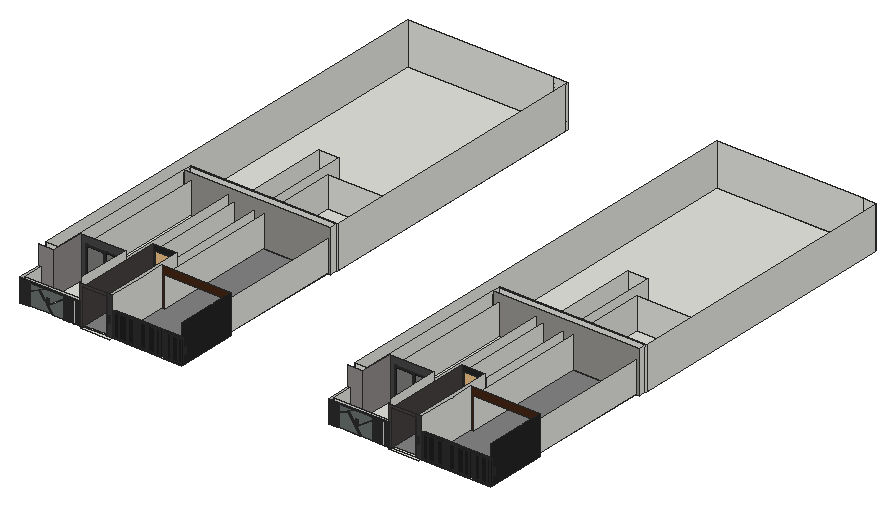
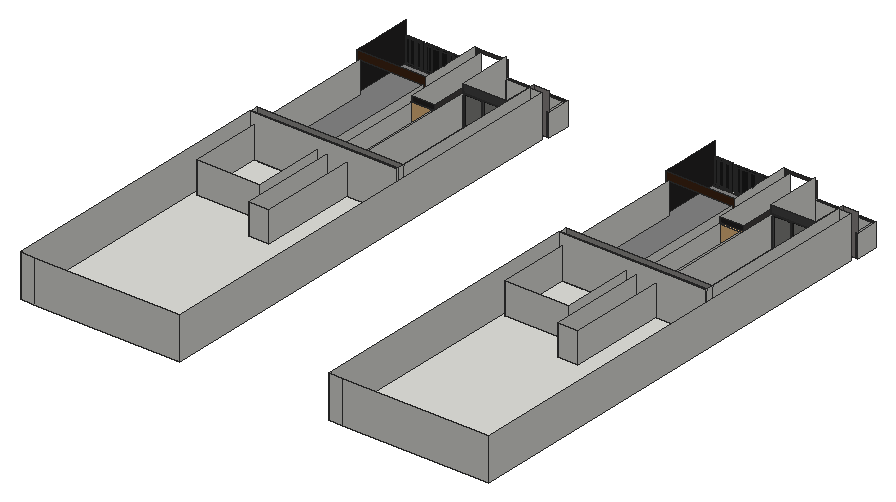
# SketchUp Ruby script. Lengths in inches.
U = 1.inch
M = Sketchup.active_model
def pt(a) = Geom::Point3d.new(a.map { |v| v * U })
def face(e, loops, mat)
  f = e.add_face(loops[0].map { |a| pt(a) })
  loops[1..].each { |l| e.add_face(l.map { |a| pt(a) }).erase! }
  f.material = f.back_material = mat if mat
  f
end
# faces: each face lists its corners as indices into pts; further lists are holes
def faces(e, pts, list, mat = nil) = list.each { |f| face(e, (f[0].is_a?(Array) ? f : [f]).map { |l| l.map { |i| pts[i] } }, mat) }
# xy, xz, yz: faces in a plane at the given z, y or x. An outline is a flat list of corners, or four numbers for a rectangle; further outlines are holes
def ring(l) = l.size == 4 ? [[l[0], l[1]], [l[2], l[1]], [l[2], l[3]], [l[0], l[3]]] : l.each_slice(2).to_a
def flat(e, list, mat, &to3) = list.each { |f| face(e, (f[0].is_a?(Array) ? f : [f]).map { |l| ring(l).map { |u, v| to3.(u, v) } }, mat) }
def xy(e, z, list, mat = nil) = flat(e, list, mat) { |x, y| [x, y, z] }
def xz(e, y, list, mat = nil) = flat(e, list, mat) { |x, z| [x, y, z] }
def yz(e, x, list, mat = nil) = flat(e, list, mat) { |y, z| [x, y, z] }
def lines(e, pts, list) = list.each { |a, b| e.add_line(pt(pts[a]), pt(pts[b])) }
# prism: a flat outline (further loops are holes) pulled along v
def prism(e, loops, v, mat = nil)
  f = face(e, loops, mat); d = Geom::Vector3d.new(v.map { |x| x * U })
  f.pushpull(f.normal.samedirection?(d) ? d.length : -d.length)
end
def box(e, o, s, mat = nil) = prism(e, [[o, [o[0] + s[0], o[1], o[2]], [o[0] + s[0], o[1] + s[1], o[2]], [o[0], o[1] + s[1], o[2]]]], [0, 0, s[2]], mat)
def at(x, y, z, deg = 0) = Geom::Transformation.translation(pt([x, y, z])) * Geom::Transformation.rotation(ORIGIN, Z_AXIS, deg.degrees)
def axes(o, x, y, z) = Geom::Transformation.new([*x, 0, *y, 0, *z, 0, *pt(o).to_a, 1])
def part(name) = M.definitions.add(name)
# library, detail: a bought-in or finely detailed component or shape, given as its bounding box
def library(name, o, s) = part(name).tap { |d| box(d.entities, o, s) }
def detail(e, o, s) = box(e.add_group.entities, o, s)
def put(e, d, t, mat = nil) = e.add_instance(d, t).tap { |i| i.material = mat if mat }
def group(e, t, mat = nil) = e.add_group.tap { |g| g.transformation = t; g.material = mat if mat }.entities
root = M.entities
M.materials.add("Glass_Tinted_Gray").color = [0, 0, 0]
M.materials["Glass_Tinted_Gray"].alpha = 0.125
M.materials.add("[0135_DarkGray]").color = [81, 81, 81]
M.materials.add("[Color M07]").color = [58, 58, 58]
M.materials.add("[Color M08]").color = [30, 30, 30]
M.materials.add("[Granite Dark Gray]").color = [38, 37, 37]
M.materials.add("[Granite Dark Gray]1").color = [69, 68, 68]
M.materials.add("[Granite Light Gray]").color = [149, 148, 144]
M.materials.add("[Granite Tile]1").color = [68, 65, 63]
M.materials.add("[Mirror 02]").color = [229, 229, 229]
M.materials.add("[Slate]").color = [102, 110, 108]
M.materials.add("[Stone Marble]").color = [143, 138, 136]
M.materials.add("[Terrazzo Light Blue]").color = [196, 214, 227]
M.materials.add("[Tile Grey]").color = [132, 132, 132]
M.materials.add("[Wood Veneer 01]").color = [66, 38, 20]
c1 = part("Group\#7")
xy(c1.entities,0,[[6,0,4.45,0.2,3,0.8,1.76,1.76,0.8,3,0.2,4.45,0,6,0.2,7.55,0.8,9,1.76,10.24,3,11.2,4.45,11.8,6,12,7.55,11.8,9,11.2,10.24,10.24,11.2,9,11.8,7.55,12,6,11.8,4.45,11.2,3,10.24,1.76,9,0.8,7.55,0.2]])
xy(c1.entities,37,[[6,0,7.55,0.2,9,0.8,10.24,1.76,11.2,3,11.8,4.45,12,6,11.8,7.55,11.2,9,10.24,10.24,9,11.2,7.55,11.8,6,12,4.45,11.8,3,11.2,1.76,10.24,0.8,9,0.2,7.55,0,6,0.2,4.45,0.8,3,1.76,1.76,3,0.8,4.45,0.2]],"[Granite Tile]1")
p = [[4.45,0.2,0],[6,0,0],[6,0,37],[4.45,0.2,37],[7.55,0.2,0],[7.55,0.2,37],
  [3,0.8,0],[3,0.8,37],[9,0.8,0],[9,0.8,37],[1.76,1.76,0],[1.76,1.76,37],
  [10.24,1.76,0],[10.24,1.76,37],[0.8,3,0],[0.8,3,37],[11.2,3,0],[11.2,3,37],
  [0.2,4.45,0],[0.2,4.45,37],[11.8,4.45,0],[11.8,4.45,37],[0,6,0],[0,6,37],
  [12,6,0],[12,6,37],[0.2,7.55,0],[0.2,7.55,37],[11.8,7.55,0],[11.8,7.55,37],
  [0.8,9,0],[0.8,9,37],[11.2,9,0],[11.2,9,37],[1.76,10.24,0],[1.76,10.24,37],
  [10.24,10.24,0],[10.24,10.24,37],[3,11.2,0],[3,11.2,37],[9,11.2,0],[9,11.2,37],
  [4.45,11.8,0],[4.45,11.8,37],[7.55,11.8,0],[7.55,11.8,37],[6,12,0],[6,12,37]]
faces(c1.entities,p,[[0,1,2,3],[1,4,5,2],[6,0,3,7],[4,8,9,5],[10,6,7,11],[8,12,13,9],[14,10,11,15],[12,16,17,13],
  [18,14,15,19],[16,20,21,17],[22,18,19,23],[20,24,25,21],[26,22,23,27],[24,28,29,25],[30,26,27,31],[28,32,33,29],
  [34,30,31,35],[32,36,37,33],[38,34,35,39],[36,40,41,37],[42,38,39,43],[40,44,45,41],[46,42,43,47],[44,46,47,45]],"[Granite Tile]1")
c2 = part("PENTEK_RP Fineline 50S_Sliding_DoorCase_E1")
box(c2.entities,[0,0,0],[1.51,3.66,99.27],"[0135_DarkGray]")
c3 = part("PENTEK_RP Fineline 50S_SlidingDooe_Case_E2")
box(c3.entities,[0,0,0],[96.25,3.66,1.51],"[0135_DarkGray]")
c4 = part("pentek_RP Fineline 50S_SlidingDoor_Case")
put(c4.entities,c2,at(97.76,0,0))
put(c4.entities,c3,at(1.51,0,0))
put(c4.entities,c2,at(0,0,0))
put(c4.entities,c3,at(1.51,0,97.76))
c5 = part("PENTEK_RP Fineline 50S_SlidingDoor_GlazingBead_2")
box(c5.entities,[0,0,0],[0.56,0.59,94.39],"[0135_DarkGray]")
c6 = part("PENTEK_RP Fineline 50S_SlidingDoor_Glass")
box(c6.entities,[0,0,0],[46.58,0.16,94.39],"Glass_Tinted_Gray")
c7 = part("PENTEK_RP Fineline 50S_SlidingDoor_GlazingBead")
box(c7.entities,[0,0,0],[45.47,0.59,0.56],"[0135_DarkGray]")
c8 = part("PENTEK_RP Fineline 50S_SlidingDoor_Leaf_E1")
xy(c8.entities,0,[[0,0,0.93,1.97],[0.93,1.57,1.49,1.97]],"[0135_DarkGray]")
xy(c8.entities,96.25,[[0,0,0.93,0,0.93,1.57,1.49,1.57,1.49,1.97,0,1.97]],"[0135_DarkGray]")
xz(c8.entities,0,[[0,0,0.93,96.25]],"[0135_DarkGray]")
xz(c8.entities,1.57,[[0.93,0,1.49,95.32],[0.93,95.32,1.49,96.25]],"[0135_DarkGray]")
xz(c8.entities,1.97,[[0,0,1.49,96.25]],"[0135_DarkGray]")
yz(c8.entities,0,[[0,0,1.97,96.25]],"[0135_DarkGray]")
yz(c8.entities,0.93,[[0,0,1.57,0.93],[0,0.93,1.57,95.32],[0,95.32,1.57,96.25]],"[0135_DarkGray]")
yz(c8.entities,1.49,[[1.57,0,1.97,95.32],[1.57,95.32,1.97,96.25]],"[0135_DarkGray]")
c9 = part("PENTEK_RP Fineline 50S_SlidingDoor_Leaf_E2")
xy(c9.entities,0,[[0,0,0,1.57,0.56,1.57,0.56,1.97,46.02,1.97,46.02,1.57,46.58,1.57,46.58,0]],"[0135_DarkGray]")
xy(c9.entities,0.93,[[0,0,46.58,1.57]],"[0135_DarkGray]")
xy(c9.entities,1.49,[[0.56,1.57,46.02,1.97]],"[0135_DarkGray]")
xz(c9.entities,0,[[0,0,46.58,0.93]],"[0135_DarkGray]")
xz(c9.entities,1.57,[[0,0,0.56,0.93],[46.02,0,46.58,0.93],[0.56,0.93,46.02,1.49]],"[0135_DarkGray]")
xz(c9.entities,1.97,[[0.56,0,46.02,1.49]],"[0135_DarkGray]")
yz(c9.entities,0,[[0,0,1.57,0.93]],"[0135_DarkGray]")
yz(c9.entities,0.56,[[1.57,0,1.97,0.93],[1.57,0.93,1.97,1.49]],"[0135_DarkGray]")
yz(c9.entities,46.02,[[1.57,0,1.97,0.93],[1.57,0.93,1.97,1.49]],"[0135_DarkGray]")
yz(c9.entities,46.58,[[0,0,1.57,0.93]],"[0135_DarkGray]")
c10 = part("PENTEK_RP Fineline S_SlidingDoor_Leaf1")
put(c10.entities,c5,at(0.93,0,0.93))
put(c10.entities,c5,at(46.96,0,0.93))
put(c10.entities,c6,at(1.49,1.42,0.93))
put(c10.entities,c7,at(1.49,0,0.93))
put(c10.entities,c6,at(1.49,0.59,0.93),"[Terrazzo Light Blue]")
put(c10.entities,c8,at(0,0,0))
put(c10.entities,c8,axes([48.44,0,0],[-1,0,0],[0,1,0],[0,0,1]))
put(c10.entities,c9,axes([0.93,0,96.25],[1,0,0],[0,1,0],[0,0,-1]))
put(c10.entities,c9,at(0.93,0,0))
put(c10.entities,c7,at(1.49,0,94.77))
c11 = part("PENTEK_RP Fineline 50S_SlidingDoor_Leaf2")
put(c11.entities,c6,at(1.49,1.42,0.93))
put(c11.entities,c7,at(1.49,0,94.77))
put(c11.entities,c5,at(46.96,0,0.93))
put(c11.entities,c6,at(1.49,0.59,0.93),"[Mirror 02]")
put(c11.entities,c5,at(0.93,0,0.93))
put(c11.entities,c8,at(0,0,0))
put(c11.entities,c8,axes([48.44,0,0],[-1,0,0],[0,1,0],[0,0,1]))
put(c11.entities,c7,at(1.49,0,0.93))
put(c11.entities,c9,axes([0.93,0,96.25],[1,0,0],[0,1,0],[0,0,-1]))
put(c11.entities,c9,at(0.93,0,0))
c12 = part("PENTEK - Slimmest Steel Sliding Door / Window\#1")
put(c12.entities,c4,at(0,-1.88,-0.09))
put(c12.entities,c10,at(1.51,-2.27,1.42))
put(c12.entities,c11,at(49.32,-0.3,1.42))
c13 = library("元件\#5",[-4.39,0,0],[5.37,35.83,90.55])
c14 = part("Group\#102")
g1 = group(c14.entities,at(0,0,0))
prism(g1,[[[0,3,72],[70.5,3,72],[70.5,3,0],[0,3,0]],[[67.5,3,3],[67.5,3,69],[3,3,69],[3,3,3]]],[0,-3,0])
c15 = part("Group\#135")
box(c15.entities,[0,0,0],[0.5,1,66])
c16 = part("Group\#148")
box(c16.entities,[0,-1,0],[5.5,1,66])
box(c16.entities,[50.84,-1,0],[13.66,1,66])
box(c16.entities,[28.06,-1,0],[22.28,1,66])
box(c16.entities,[24.66,-1,0],[2.9,1,66])
box(c16.entities,[6,-1,0],[18.16,1,66])
c17 = part("Component\#23")
g2 = group(c17.entities,at(70.5,0,0),"[Color M08]")
put(g2,c14,axes([70.5,0,0],[-1,0,0],[0,1,0],[0,0,1]))
g3 = group(g2,at(3,2,3))
g4 = group(g3,at(0,-1,0))
box(g4,[0,0,0],[5.5,1,66])
box(g4,[50.84,0,0],[13.66,1,66])
box(g4,[28.06,0,0],[22.28,1,66])
box(g4,[24.66,0,0],[2.9,1,66])
box(g4,[6,0,0],[18.16,1,66])
put(g3,c15,axes([50.34,0,0],[1,0,0],[0,-1,0],[0,0,1]))
put(g3,c15,axes([24.16,0,0],[1,0,0],[0,-1,0],[0,0,1]))
put(g3,c15,axes([27.56,0,0],[1,0,0],[0,-1,0],[0,0,1]))
put(g3,c15,axes([5.5,0,0],[1,0,0],[0,-1,0],[0,0,1]))
g5 = group(c17.entities,at(70.5,0,0),"[Color M08]")
put(g5,c14,at(-70.5,0,0))
g6 = group(g5,at(-3,2,3,-180))
put(g6,c16,at(0,1,0))
put(g6,c15,at(50.34,0,0))
put(g6,c15,at(24.16,0,0))
put(g6,c15,at(27.56,0,0))
put(g6,c15,at(5.5,0,0))
g7 = group(c17.entities,at(150,0,0),"[Color M08]")
put(g7,c14,axes([54,0,0],[-0.76596,0,0],[0,1,0],[0,0,1]))
g8 = group(g7,at(2.3,2,3))
put(g8,c16,axes([0,-1,0],[0.76596,0,0],[0,-1,0],[0,0,1]))
put(g8,c15,axes([38.55,0,0],[0.76596,0,0],[0,-1,0],[0,0,1]))
put(g8,c15,axes([18.5,0,0],[0.76596,0,0],[0,-1,0],[0,0,1]))
put(g8,c15,axes([21.11,0,0],[0.76596,0,0],[0,-1,0],[0,0,1]))
put(g8,c15,axes([4.22,0,0],[0.76596,0,0],[0,-1,0],[0,0,1]))
xy(root,8.5,[[395.95,450,480.15,458.5],[1274.7,450,1358.9,458.5],[218.97,457.5625,222.53,458.5],[223.78,457.5625,227.34,458.5],[228.6,457.5625,232.16,458.5],
  [233.41,457.5625,236.97,458.5],[238.22,457.5625,241.78,458.5],[243.03,457.5625,246.59,458.5],[343.47,457.5625,347.43,458.5],[348.47,457.5625,352.43,458.5],
  [353.47,457.5625,357.43,458.5],[358.47,457.5625,362.43,458.5],[363.47,457.5625,367.43,458.5],[368.47,457.5625,372.43,458.5],[378.2,457.5625,381.86,458.5],
  [385.66,457.5625,388.78,458.5],[1097.72,457.5625,1101.28,458.5],[1102.53,457.5625,1106.09,458.5],[1107.35,457.5625,1110.91,458.5],[1112.16,457.5625,1115.72,458.5],
  [1116.97,457.5625,1120.53,458.5],[1121.78,457.5625,1125.34,458.5],[1222.22,457.5625,1226.18,458.5],[1227.22,457.5625,1231.18,458.5],[1232.22,457.5625,1236.18,458.5],
  [1237.22,457.5625,1241.18,458.5],[1242.22,457.5625,1246.18,458.5],[1247.22,457.5625,1251.18,458.5],[1256.95,457.5625,1260.61,458.5],[1264.41,457.5625,1267.53,458.5],
  [218.97,458.5,218.97,523.18,225.79,523.18,225.79,465.32,388.78,465.32,388.78,458.5,310.12,458.5,310.12,461.375,306.57,461.375,306.57,458.5],[306.57,458.5,310.12,461.375],[395.95,458.5,463.7,465.32],[481.29,458.5,678.9,465.32],[1097.72,458.5,1097.72,523.18,1104.54,523.18,1104.54,465.32,1267.53,465.32,1267.53,458.5,1188.87,458.5,1188.87,461.375,1185.32,461.375,1185.32,458.5],
  [1185.32,458.5,1188.87,461.375],[1274.7,458.5,1342.45,465.32],[1360.04,458.5,1557.65,465.32],[225.79,465.32,388.78,465.32,388.78,619.06,262.66,619.06,262.66,523.18,225.79,523.18],[1104.54,465.32,1267.53,465.32,1267.53,619.06,1141.41,619.06,1141.41,523.18,1104.54,523.18],
  [225.79,539.02,261.53,539.02,261.53,1010.9,402.97,1010.9,402.97,1288.43,460.85,1288.43,460.85,1010.9,488.9,1010.9,488.9,1213.68,669.8,1213.68,669.8,1010.9,678.9,1010.9,678.9,1828.81,225.79,1828.81],[1104.54,539.02,1140.28,539.02,1140.28,1010.9,1281.72,1010.9,1281.72,1288.43,1339.6,1288.43,1339.6,1010.9,1367.65,1010.9,1367.65,1213.68,1548.55,1213.68,1548.55,1010.9,1557.65,1010.9,1557.65,1828.81,1104.54,1828.81],[261.53,986.46,402.97,1006.15],[402.97,986.46,460.85,1006.15],[460.85,986.46,488.9,1006.15],
  [488.9,986.46,669.8,1006.15],[669.8,986.46,678.9,1006.15],[1140.28,986.46,1281.72,1006.15],[1281.72,986.46,1339.6,1006.15],[1339.6,986.46,1367.65,1006.15],
  [1367.65,986.46,1548.55,1006.15],[1548.55,986.46,1557.65,1006.15],[261.53,1006.15,402.97,1010.9],[402.97,1006.15,460.85,1010.9],[460.85,1006.15,488.9,1010.9],
  [488.9,1006.15,669.8,1010.9],[669.8,1006.15,678.9,1010.9],[1140.28,1006.15,1281.72,1010.9],[1281.72,1006.15,1339.6,1010.9],[1339.6,1006.15,1367.65,1010.9],
  [1367.65,1006.15,1548.55,1010.9],[1548.55,1006.15,1557.65,1010.9],[402.97,1010.9,460.85,1288.43],[488.9,1010.9,669.8,1213.68],[1281.72,1010.9,1339.6,1288.43],
  [1367.65,1010.9,1548.55,1213.68]])
xy(root,8.5,[[395.95,465.32,463.7,465.32,463.7,706.62,460.85,706.62,460.85,986.46,402.97,986.46,402.97,706.62,395.95,706.62],[481.29,465.32,678.9,465.32,678.9,633.06,669.8,633.06,669.8,986.46,488.9,986.46,488.9,633.06,481.29,633.06],[1274.7,465.32,1342.45,465.32,1342.45,706.62,1339.6,706.62,1339.6,986.46,1281.72,986.46,1281.72,706.62,1274.7,706.62],[1360.04,465.32,1557.65,465.32,1557.65,633.06,1548.55,633.06,1548.55,986.46,1367.65,986.46,1367.65,633.06,1360.04,633.06]],"[Tile Grey]")
xy(root,20.01,[[279.88,619.06,385.01,1006.15],[1158.63,619.06,1263.76,1006.15]])
xy(root,68.78,[[222.53,457.5625,223.78,458.5],[227.34,457.5625,228.6,458.5],[232.16,457.5625,233.41,458.5],[236.97,457.5625,238.22,458.5],[241.78,457.5625,243.03,458.5],
  [246.59,457.5625,246.59,458.5,290.35,458.5,290.35,461.375,293.48,461.375,293.48,458.5,343.47,458.5,343.47,457.5625],[347.43,457.5625,348.47,458.5],[352.43,457.5625,353.47,458.5],[357.43,457.5625,358.47,458.5],[362.43,457.5625,363.47,458.5],
  [367.43,457.5625,368.47,458.5],[372.43,457.5625,378.2,458.5],[381.86,457.5625,385.66,458.5],[1101.28,457.5625,1102.53,458.5],[1106.09,457.5625,1107.35,458.5],
  [1110.91,457.5625,1112.16,458.5],[1115.72,457.5625,1116.97,458.5],[1120.53,457.5625,1121.78,458.5],[1125.34,457.5625,1125.34,458.5,1169.1,458.5,1169.1,461.375,1172.23,461.375,1172.23,458.5,1222.22,458.5,1222.22,457.5625],[1226.18,457.5625,1227.22,458.5],
  [1231.18,457.5625,1232.22,458.5],[1236.18,457.5625,1237.22,458.5],[1241.18,457.5625,1242.22,458.5],[1246.18,457.5625,1247.22,458.5],[1251.18,457.5625,1256.95,458.5],
  [1260.61,457.5625,1264.41,458.5]])
xz(root,457.5625,[[218.97,8.5,222.53,68.78],[223.78,8.5,227.34,68.78],[228.6,8.5,232.16,68.78],[233.41,8.5,236.97,68.78],[238.22,8.5,241.78,68.78],
  [243.03,8.5,246.59,68.78],[343.47,8.5,347.43,68.78],[348.47,8.5,352.43,68.78],[353.47,8.5,357.43,68.78],[358.47,8.5,362.43,68.78],
  [363.47,8.5,367.43,68.78],[385.66,8.5,388.78,68.78],[1097.72,8.5,1101.28,68.78],[1102.53,8.5,1106.09,68.78],[1107.35,8.5,1110.91,68.78],
  [1112.16,8.5,1115.72,68.78],[1116.97,8.5,1120.53,68.78],[1121.78,8.5,1125.34,68.78],[1222.22,8.5,1226.18,68.78],[1227.22,8.5,1231.18,68.78],
  [1232.22,8.5,1236.18,68.78],[1237.22,8.5,1241.18,68.78],[1242.22,8.5,1246.18,68.78],[1264.41,8.5,1267.53,68.78],[218.97,68.78,388.78,72.4375],
  [1097.72,68.78,1267.53,72.4375]],"[Color M08]")
xz(root,457.5625,[[368.47,8.5,372.43,68.78],[378.2,8.5,381.86,68.78],[1247.22,8.5,1251.18,68.78],[1256.95,8.5,1260.61,68.78]],"[Slate]")
xz(root,458.5,[[222.53,8.5,223.78,68.78],[227.34,8.5,228.6,68.78],[232.16,8.5,233.41,68.78],[236.97,8.5,238.22,68.78],[241.78,8.5,243.03,68.78],
  [347.43,8.5,348.47,68.78],[352.43,8.5,353.47,68.78],[357.43,8.5,358.47,68.78],[362.43,8.5,363.47,68.78],[367.43,8.5,368.47,68.78],
  [1101.28,8.5,1102.53,68.78],[1106.09,8.5,1107.35,68.78],[1110.91,8.5,1112.16,68.78],[1115.72,8.5,1116.97,68.78],[1120.53,8.5,1121.78,68.78],
  [1226.18,8.5,1227.22,68.78],[1231.18,8.5,1232.22,68.78],[1236.18,8.5,1237.22,68.78],[1241.18,8.5,1242.22,68.78],[1246.18,8.5,1247.22,68.78]])
xz(root,458.5,[[463.7,8.5,481.29,118.38],[1342.45,8.5,1360.04,118.38]],"[Color M07]")
xz(root,458.5,[[372.43,8.5,378.2,68.78],[381.86,8.5,385.66,68.78],[1251.18,8.5,1256.95,68.78],[1260.61,8.5,1264.41,68.78]],"[Color M08]")
xz(root,458.5,[[388.78,8.5,395.95,8.5,395.95,110.32,463.7,110.32,463.7,118.38,388.78,118.38],[1267.53,8.5,1274.7,8.5,1274.7,110.32,1342.45,110.32,1342.45,118.38,1267.53,118.38]],"[Granite Tile]1")
xz(root,458.5,[[246.59,8.5,306.57,8.5,271.87,57.375,246.59,44.04],[310.12,8.5,343.47,8.5,343.47,58.8,297.81,25.91],[1125.34,8.5,1185.32,8.5,1150.62,57.375,1125.34,44.04],[1188.87,8.5,1222.22,8.5,1222.22,58.8,1176.56,25.91],[295.39,29.34,343.47,62.06,343.47,68.78,293.48,68.78,274.57,58.8],
  [1174.14,29.34,1222.22,62.06,1222.22,68.78,1172.23,68.78,1153.32,58.8],[246.59,46.32,290.35,68.78,246.59,68.78],[1125.34,46.32,1169.1,68.78,1125.34,68.78]],"[Slate]")
xz(root,461.375,[[306.57,8.5,310.12,8.5,297.81,25.91,295.39,29.34,274.57,58.8,271.87,57.375],[1185.32,8.5,1188.87,8.5,1176.56,25.91,1174.14,29.34,1153.32,58.8,1150.62,57.375],[297.81,25.91,343.47,58.8,343.47,62.06,295.39,29.34],[1176.56,25.91,1222.22,58.8,1222.22,62.06,1174.14,29.34],[246.59,44.04,271.87,57.375,274.57,58.8,293.48,68.78,290.35,68.78,246.59,46.32],
  [1125.34,44.04,1150.62,57.375,1153.32,58.8,1172.23,68.78,1169.1,68.78,1125.34,46.32]])
xz(root,465.32,[[225.79,8.5,388.78,72.4375],[1104.54,8.5,1267.53,72.4375]])
xz(root,523.18,[[218.97,8.5,225.79,72.4375],[1097.72,8.5,1104.54,72.4375]])
xz(root,523.18,[[225.79,8.5,262.66,8.5,262.66,128.5,218.97,128.5,218.97,72.4375,225.79,72.4375],[1104.54,8.5,1141.41,8.5,1141.41,128.5,1097.72,128.5,1097.72,72.4375,1104.54,72.4375]],"[Stone Marble]")
xz(root,539.02,[[225.79,8.5,261.53,128.5],[1104.54,8.5,1140.28,128.5]])
xz(root,619.06,[[[262.66,8.5,388.78,128.5],[279.88,20.01,385.01,107.07]],[[1141.41,8.5,1267.53,128.5],[1158.63,20.01,1263.76,107.07]]],"[Granite Dark Gray]1")
xz(root,633.06,[[481.29,8.5,488.9,8.5,488.9,96.29,669.8,96.29,669.8,8.5,678.9,8.5,678.9,118.38,481.29,118.38],[1360.04,8.5,1367.65,8.5,1367.65,96.29,1548.55,96.29,1548.55,8.5,1557.65,8.5,1557.65,118.38,1360.04,118.38]],"[Wood Veneer 01]")
xz(root,706.62,[[395.95,8.5,402.97,8.5,402.97,96.1875,460.85,96.1875,460.85,8.5,463.7,8.5,463.7,110.32,395.95,110.32],[1274.7,8.5,1281.72,8.5,1281.72,96.1875,1339.6,96.1875,1339.6,8.5,1342.45,8.5,1342.45,110.32,1274.7,110.32]],"[Granite Dark Gray]")
xz(root,986.46,[[261.53,8.5,678.9,128.5],[1140.28,8.5,1557.65,128.5]],"[Granite Light Gray]")
xz(root,1006.15,[[[261.53,8.5,678.9,128.5],[279.88,20.01,385.01,107.07]],[[1140.28,8.5,1557.65,128.5],[1158.63,20.01,1263.76,107.07]]])
xz(root,1010.9,[[261.53,8.5,678.9,128.5],[1140.28,8.5,1557.65,128.5]])
xz(root,1213.68,[[488.9,8.5,669.8,96.29],[1367.65,8.5,1548.55,96.29]])
xz(root,1288.43,[[402.97,8.5,460.85,96.1875],[1281.72,8.5,1339.6,96.1875]])
xz(root,1828.81,[[225.79,8.5,640.4,128.5],[640.4,8.5,678.9,128.5],[1104.54,8.5,1519.15,128.5],[1519.15,8.5,1557.65,128.5]])
yz(root,218.97,[[457.5625,8.5,523.18,72.4375]])
yz(root,222.53,[[457.5625,8.5,458.5,68.78]])
yz(root,223.78,[[457.5625,8.5,458.5,68.78]])
yz(root,225.79,[[465.32,8.5,523.18,72.4375],[539.02,8.5,1828.81,128.5]])
yz(root,227.34,[[457.5625,8.5,458.5,68.78]])
yz(root,228.6,[[457.5625,8.5,458.5,68.78]])
yz(root,232.16,[[457.5625,8.5,458.5,68.78]])
yz(root,233.41,[[457.5625,8.5,458.5,68.78]])
yz(root,236.97,[[457.5625,8.5,458.5,68.78]])
yz(root,238.22,[[457.5625,8.5,458.5,68.78]])
yz(root,241.78,[[457.5625,8.5,458.5,68.78]])
yz(root,243.03,[[457.5625,8.5,458.5,68.78]])
yz(root,246.59,[[457.5625,8.5,458.5,8.5,458.5,44.04,461.375,44.04,461.375,46.32,458.5,46.32,458.5,68.78,457.5625,68.78]])
yz(root,261.53,[[539.02,8.5,986.46,128.5],[986.46,8.5,1006.15,128.5],[1006.15,8.5,1010.9,128.5]])
yz(root,262.66,[[523.18,8.5,619.06,128.5]],"[Stone Marble]")
yz(root,279.88,[[619.06,20.01,1006.15,107.07]])
yz(root,343.47,[[457.5625,8.5,457.5625,68.78,458.5,68.78,458.5,62.06,461.375,62.06,461.375,58.8,458.5,58.8,458.5,8.5]])
yz(root,347.43,[[457.5625,8.5,458.5,68.78]])
yz(root,348.47,[[457.5625,8.5,458.5,68.78]])
yz(root,352.43,[[457.5625,8.5,458.5,68.78]])
yz(root,353.47,[[457.5625,8.5,458.5,68.78]])
yz(root,357.43,[[457.5625,8.5,458.5,68.78]])
yz(root,358.47,[[457.5625,8.5,458.5,68.78]])
yz(root,362.43,[[457.5625,8.5,458.5,68.78]])
yz(root,363.47,[[457.5625,8.5,458.5,68.78]])
yz(root,367.43,[[457.5625,8.5,458.5,68.78]])
yz(root,368.47,[[457.5625,8.5,458.5,68.78]])
yz(root,372.43,[[457.5625,8.5,458.5,68.78]])
yz(root,378.2,[[457.5625,8.5,458.5,68.78]])
yz(root,381.86,[[457.5625,8.5,458.5,68.78]])
yz(root,385.01,[[619.06,20.01,1006.15,107.07]])
yz(root,385.66,[[457.5625,8.5,458.5,68.78]])
yz(root,388.78,[[457.5625,8.5,458.5,68.78],[458.5,8.5,465.32,72.4375],[465.32,8.5,619.06,128.5],[457.5625,68.78,458.5,72.4375]])
yz(root,395.95,[[458.5,8.5,706.62,110.32]],"[Granite Tile]1")
yz(root,402.97,[[706.62,8.5,1288.43,96.1875]])
yz(root,460.85,[[706.62,8.5,1288.43,96.1875]])
yz(root,463.7,[[458.5,8.5,706.62,110.32]])
yz(root,481.29,[[458.5,8.5,633.06,8.5,633.06,118.38,571.64,118.38,571.64,116.94,561.06,116.94,561.06,118.38,458.5,118.38]])
yz(root,488.9,[[633.06,8.5,1213.68,96.29]])
yz(root,669.8,[[633.06,8.5,1213.68,96.29]])
yz(root,678.9,[[986.46,8.5,1006.15,128.5],[1006.15,8.5,1010.9,128.5],[1010.9,8.5,1822.82,128.5],[1822.82,8.5,1828.81,128.5]])
yz(root,678.9,[[458.5,8.5,458.5,118.38,561.06,118.38,561.06,116.94,571.64,116.94,571.64,118.38,633.06,118.38,633.06,8.5]],"[Granite Dark Gray]")
yz(root,1097.72,[[457.5625,8.5,523.18,72.4375]])
yz(root,1101.28,[[457.5625,8.5,458.5,68.78]])
yz(root,1102.53,[[457.5625,8.5,458.5,68.78]])
yz(root,1104.54,[[465.32,8.5,523.18,72.4375],[539.02,8.5,1828.81,128.5]])
yz(root,1106.09,[[457.5625,8.5,458.5,68.78]])
yz(root,1107.35,[[457.5625,8.5,458.5,68.78]])
yz(root,1110.91,[[457.5625,8.5,458.5,68.78]])
yz(root,1112.16,[[457.5625,8.5,458.5,68.78]])
yz(root,1115.72,[[457.5625,8.5,458.5,68.78]])
yz(root,1116.97,[[457.5625,8.5,458.5,68.78]])
yz(root,1120.53,[[457.5625,8.5,458.5,68.78]])
yz(root,1121.78,[[457.5625,8.5,458.5,68.78]])
yz(root,1125.34,[[457.5625,8.5,458.5,8.5,458.5,44.04,461.375,44.04,461.375,46.32,458.5,46.32,458.5,68.78,457.5625,68.78]])
yz(root,1140.28,[[539.02,8.5,986.46,128.5],[986.46,8.5,1006.15,128.5],[1006.15,8.5,1010.9,128.5]])
yz(root,1141.41,[[523.18,8.5,619.06,128.5]],"[Stone Marble]")
yz(root,1158.63,[[619.06,20.01,1006.15,107.07]])
yz(root,1222.22,[[457.5625,8.5,457.5625,68.78,458.5,68.78,458.5,62.06,461.375,62.06,461.375,58.8,458.5,58.8,458.5,8.5]])
yz(root,1226.18,[[457.5625,8.5,458.5,68.78]])
yz(root,1227.22,[[457.5625,8.5,458.5,68.78]])
yz(root,1231.18,[[457.5625,8.5,458.5,68.78]])
yz(root,1232.22,[[457.5625,8.5,458.5,68.78]])
yz(root,1236.18,[[457.5625,8.5,458.5,68.78]])
yz(root,1237.22,[[457.5625,8.5,458.5,68.78]])
yz(root,1241.18,[[457.5625,8.5,458.5,68.78]])
yz(root,1242.22,[[457.5625,8.5,458.5,68.78]])
yz(root,1246.18,[[457.5625,8.5,458.5,68.78]])
yz(root,1247.22,[[457.5625,8.5,458.5,68.78]])
yz(root,1251.18,[[457.5625,8.5,458.5,68.78]])
yz(root,1256.95,[[457.5625,8.5,458.5,68.78]])
yz(root,1260.61,[[457.5625,8.5,458.5,68.78]])
yz(root,1263.76,[[619.06,20.01,1006.15,107.07]])
yz(root,1264.41,[[457.5625,8.5,458.5,68.78]])
yz(root,1267.53,[[457.5625,8.5,458.5,68.78],[458.5,8.5,465.32,72.4375],[465.32,8.5,619.06,128.5],[457.5625,68.78,458.5,72.4375]])
yz(root,1274.7,[[458.5,8.5,706.62,110.32]],"[Granite Tile]1")
yz(root,1281.72,[[706.62,8.5,1288.43,96.1875]])
yz(root,1339.6,[[706.62,8.5,1288.43,96.1875]])
yz(root,1342.45,[[458.5,8.5,706.62,110.32]])
yz(root,1360.04,[[458.5,8.5,633.06,8.5,633.06,118.38,571.64,118.38,571.64,116.94,561.06,116.94,561.06,118.38,458.5,118.38]])
yz(root,1367.65,[[633.06,8.5,1213.68,96.29]])
yz(root,1548.55,[[633.06,8.5,1213.68,96.29]])
yz(root,1557.65,[[986.46,8.5,1006.15,128.5],[1006.15,8.5,1010.9,128.5],[1010.9,8.5,1822.82,128.5],[1822.82,8.5,1828.81,128.5]])
yz(root,1557.65,[[458.5,8.5,458.5,118.38,561.06,118.38,561.06,116.94,571.64,116.94,571.64,118.38,633.06,118.38,633.06,8.5]],"[Granite Dark Gray]")
p = [[271.87,458.5,57.375],[306.57,458.5,8.5],[306.57,461.375,8.5],[271.87,461.375,57.375],[310.12,458.5,8.5],[297.81,458.5,25.91],
  [297.81,461.375,25.91],[310.12,461.375,8.5],[1150.62,458.5,57.375],[1185.32,458.5,8.5],[1185.32,461.375,8.5],[1150.62,461.375,57.375],
  [1188.87,458.5,8.5],[1176.56,458.5,25.91],[1176.56,461.375,25.91],[1188.87,461.375,8.5],[343.47,458.5,58.8],[343.47,461.375,58.8],
  [1222.22,458.5,58.8],[1222.22,461.375,58.8],[295.39,458.5,29.34],[274.57,458.5,58.8],[274.57,461.375,58.8],[295.39,461.375,29.34],
  [343.47,458.5,62.06],[343.47,461.375,62.06],[1174.14,458.5,29.34],[1153.32,458.5,58.8],[1153.32,461.375,58.8],[1174.14,461.375,29.34],
  [1222.22,458.5,62.06],[1222.22,461.375,62.06],[246.59,458.5,44.04],[246.59,461.375,44.04],[1125.34,458.5,44.04],[1125.34,461.375,44.04],
  [290.35,458.5,68.78],[246.59,458.5,46.32],[246.59,461.375,46.32],[290.35,461.375,68.78],[1169.1,458.5,68.78],[1125.34,458.5,46.32],
  [1125.34,461.375,46.32],[1169.1,461.375,68.78],[293.48,458.5,68.78],[293.48,461.375,68.78],[1172.23,458.5,68.78],[1172.23,461.375,68.78]]
faces(root,p,[[0,1,2,3],[4,5,6,7],[8,9,10,11],[12,13,14,15],[5,16,17,6],[13,18,19,14],[20,21,22,23],[24,20,23,25],
  [26,27,28,29],[30,26,29,31],[32,0,3,33],[34,8,11,35],[36,37,38,39],[40,41,42,43],[21,44,45,22],[27,46,47,28]])
put(root,c1,axes([294.35,456.34,29.51],[0.42,0,0],[0,0.42,0],[0,0,0.42]))
put(root,c12,axes([276.88,619.06,20],[1.08916,0,0],[0,1,0],[0,0,0.87793]))
put(root,c13,axes([402.97,706.99,8.5],[0,-1,0],[1.61541,0,0],[0,0,0.96838]))
put(root,c1,axes([469.78,453.46,47.16],[0.42,0,0],[0,0.42,0],[0,0,0.42]))
put(root,c17,axes([481.29,458.5,8.5],[0.9687,0,0],[0,1,0],[0,0,1]))
put(root,c1,axes([685.86,453.46,44.5],[0.42,0,0],[0,0.42,0],[0,0,0.42]))
put(root,c1,axes([1173.1,456.34,29.51],[0.42,0,0],[0,0.42,0],[0,0,0.42]))
put(root,c12,axes([1155.63,619.06,20],[1.08916,0,0],[0,1,0],[0,0,0.87793]))
put(root,c13,axes([1281.72,706.99,8.5],[0,-1,0],[1.61541,0,0],[0,0,0.96838]))
put(root,c1,axes([1348.53,453.46,47.16],[0.42,0,0],[0,0.42,0],[0,0,0.42]))
put(root,c17,axes([1360.04,458.5,8.5],[0.9687,0,0],[0,1,0],[0,0,1]))
put(root,c1,axes([1564.61,453.46,44.5],[0.42,0,0],[0,0.42,0],[0,0,0.42]))
